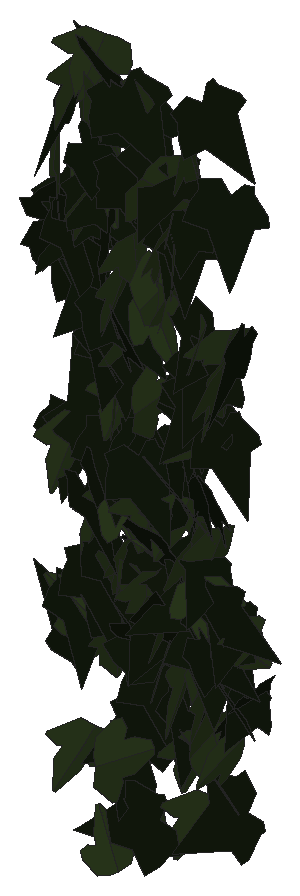
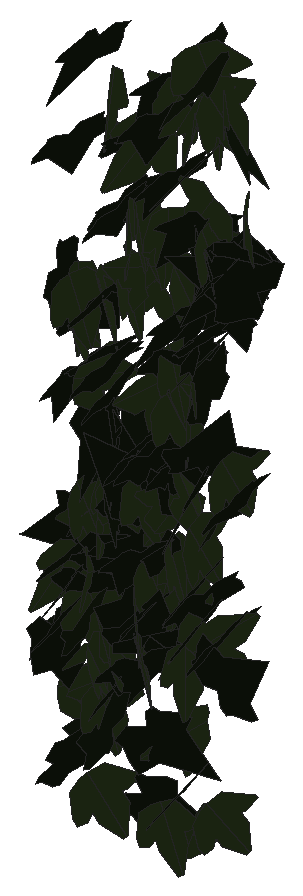
# SketchUp Ruby script. Lengths in inches.
U = 1.inch
M = Sketchup.active_model
def pt(a) = Geom::Point3d.new(a.map { |v| v * U })
def face(e, loops, mat)
  f = e.add_face(loops[0].map { |a| pt(a) })
  loops[1..].each { |l| e.add_face(l.map { |a| pt(a) }).erase! }
  f.material = f.back_material = mat if mat
  f
end
# faces: each face lists its corners as indices into pts; further lists are holes
def faces(e, pts, list, mat = nil) = list.each { |f| face(e, (f[0].is_a?(Array) ? f : [f]).map { |l| l.map { |i| pts[i] } }, mat) }
# xy, xz, yz: faces in a plane at the given z, y or x. An outline is a flat list of corners, or four numbers for a rectangle; further outlines are holes
def ring(l) = l.size == 4 ? [[l[0], l[1]], [l[2], l[1]], [l[2], l[3]], [l[0], l[3]]] : l.each_slice(2).to_a
def flat(e, list, mat, &to3) = list.each { |f| face(e, (f[0].is_a?(Array) ? f : [f]).map { |l| ring(l).map { |u, v| to3.(u, v) } }, mat) }
def xy(e, z, list, mat = nil) = flat(e, list, mat) { |x, y| [x, y, z] }
def xz(e, y, list, mat = nil) = flat(e, list, mat) { |x, z| [x, y, z] }
def yz(e, x, list, mat = nil) = flat(e, list, mat) { |y, z| [x, y, z] }
def lines(e, pts, list) = list.each { |a, b| e.add_line(pt(pts[a]), pt(pts[b])) }
# prism: a flat outline (further loops are holes) pulled along v
def prism(e, loops, v, mat = nil)
  f = face(e, loops, mat); d = Geom::Vector3d.new(v.map { |x| x * U })
  f.pushpull(f.normal.samedirection?(d) ? d.length : -d.length)
end
def box(e, o, s, mat = nil) = prism(e, [[o, [o[0] + s[0], o[1], o[2]], [o[0] + s[0], o[1] + s[1], o[2]], [o[0], o[1] + s[1], o[2]]]], [0, 0, s[2]], mat)
def at(x, y, z, deg = 0) = Geom::Transformation.translation(pt([x, y, z])) * Geom::Transformation.rotation(ORIGIN, Z_AXIS, deg.degrees)
def axes(o, x, y, z) = Geom::Transformation.new([*x, 0, *y, 0, *z, 0, *pt(o).to_a, 1])
def part(name) = M.definitions.add(name)
# library, detail: a bought-in or finely detailed component or shape, given as its bounding box
def library(name, o, s) = part(name).tap { |d| box(d.entities, o, s) }
def detail(e, o, s) = box(e.add_group.entities, o, s)
def put(e, d, t, mat = nil) = e.add_instance(d, t).tap { |i| i.material = mat if mat }
def group(e, t, mat = nil) = e.add_group.tap { |g| g.transformation = t; g.material = mat if mat }.entities
root = M.entities
M.materials.add("efeu1").color = [18, 25, 13]
M.materials.add("efeu2").color = [43, 57, 29]
c1 = part("ivyleaf_9")
p = [[1.54,2.16,1.25],[1.36,2.04,1.19],[-0.21,0.99,0.68],[-0.71,1.11,0.82],[-0.85,0.86,0.67],[-0.8,0.17,0.21],
  [-0.9,-0.01,0.1],[-0.67,-0.16,-0.02],[-0.08,-0.08,-0.05],[-0.03,-0.6,-0.4],[0.65,-0.88,-0.66],[0.83,-0.6,-0.49],
  [1.29,-0.42,-0.43],[1.8125,-0.07,-0.26],[1.21,0.44,0.15]]
faces(c1.entities,p,[[0,1,2,3,4,5,6,7,8,9,10,11,12,13,14]],"efeu1")
c2 = part("ivyleaf_10")
p = [[0,0.5,-0.03],[-0.0625,2.02,-0.43],[-0.19,2.01,-0.46],[-0.54,1.05,-0.29],[-0.52,0.625,-0.18],[-0.83,0.76,-0.28],
  [-1.16,0.64,-0.33],[-1.15,0.33,-0.24],[-0.77,-0.39,0.02],[-0.3,-0.51,0.16],[0.04,-0.48,0.23],[-0.02,2.01,-0.4375],
  [-0.06,2.01,-0.43],[0.04,-0.49,0.23],[0.67,-0.49,0.14],[1.38,0.36,-0.2],[1.375,0.51,-0.24],[0.81,0.65,-0.19],
  [0.62,0.59,-0.15],[0.6,1.09,-0.28],[0.5,1.23,-0.31]]
faces(c2.entities,p,[[0,1,2,3,4,5,6,7,8,9,10],[11,12,0,13,14,15,16,17,18,19,20]],"efeu2")
put(root,c1,axes([522.17,133.86,190.29],[0.49704,-0.38709,-0.5058],[-0.2385,0.4818,-0.60309],[0.59059,0.52034,0.18214]))
put(root,c2,axes([519.06,134.07,182.82],[0.11061,0.72226,0.03],[-0.05424,-0.02197,0.72895],[0.72084,-0.11248,0.05025]))
put(root,c2,axes([519.3,133.52,185.96],[0.08059,-0.14337,-0.86405],[0.35934,0.79672,-0.09868],[0.79875,-0.34396,0.13158]))
put(root,c2,axes([517.37,134.58,194.53],[-0.17439,-0.69901,0.42648],[0.13226,-0.45437,-0.69063],[0.80809,-0.07649,0.20507]))
put(root,c1,axes([517.86,134.49,192.92],[0.40289,-0.6896,0.17223],[0.08138,-0.15191,-0.79864],[0.70611,0.41098,-0.00622]))
put(root,c2,axes([521.91,134.17,191.51],[0.62913,0.42133,0.11867],[0.08795,0.08188,-0.75695],[-0.4288,0.63497,0.01886]))
put(root,c1,axes([519.75,134.29,194.6],[0.10741,-0.71739,-0.34234],[0.00616,0.34619,-0.72352],[0.79486,0.09426,0.05187]))
put(root,c2,axes([518.95,134.53,199.5625],[0.20121,-0.74109,0.28245],[0.09613,-0.26646,-0.76761],[0.78724,0.22195,0.02154]))
put(root,c1,axes([520.43,134.78,203.37],[-0.3338,-0.74643,0.16803],[-0.00432,-0.18148,-0.81477],[0.76509,-0.32668,0.0687]))
put(root,c1,axes([520.19,134.43,184.13],[-0.15629,-0.12747,-0.81514],[-0.62348,-0.52511,0.20166],[-0.54035,0.64277,0.00309]))
put(root,c1,axes([520.42,134.11,194.5625],[0.78632,-0.27011,-0.05779],[-0.05213,0.02613,-0.83139],[0.27126,0.78801,0.00775]))
put(root,c1,axes([517.59,134.72,189.65],[0.05804,-0.8437,0.16627],[0.01144,-0.16588,-0.84569],[0.85985,0.05916,0.00002]))
put(root,c1,axes([521.65,134.83,192.1],[-0.09761,-0.68958,0.36515],[-0.01287,-0.36653,-0.69561],[0.78019,-0.09232,0.03421]))
put(root,c1,axes([522.12,134.17,191.16],[0.13868,-0.13524,-0.79554],[0.62573,0.52773,0.01937],[0.50955,-0.61125,0.19273]))
put(root,c1,axes([517.32,134.57,204.45],[-0.60436,0.19155,-0.52821],[0.47673,-0.23575,-0.63095],[-0.29736,-0.76726,0.062]))
put(root,c1,axes([518.25,133.97,203.38],[0.56318,-0.38083,-0.47393],[-0.17077,0.52092,-0.62152],[0.5835,0.52003,0.27552]))
put(root,c1,axes([519.25,134.31,205.18],[0.0955,-0.69118,-0.44409],[0.14908,0.45424,-0.67492],[0.80791,-0.00212,0.17703]))
put(root,c2,axes([521.65,134.91,195.89],[-0.14462,-0.10083,0.78985],[0.0062,-0.80289,-0.10135],[0.79623,-0.01206,0.14425]))
put(root,c1,axes([521.81,134.81,197.78],[-0.30023,-0.71781,0.15186],[-0.03118,-0.15145,-0.77753],[0.73304,-0.30044,0.02912]))
put(root,c2,axes([518.31,134.51,206.1],[-0.63271,-0.46629,0.31865],[-0.16784,-0.30164,-0.77468],[0.53925,-0.64099,0.13275]))
put(root,c1,axes([518.4,134.875,197.22],[-0.04207,-0.69428,0.40959],[0.11743,-0.41105,-0.6847],[0.7975,0.0239,0.12243]))
put(root,c1,axes([518.49,134.6,198.14],[0.38473,-0.07551,-0.73353],[0.73566,-0.01756,0.38766],[-0.05068,-0.82812,0.05866]))
put(root,c2,axes([522.28,134.9,186.79],[0.00844,-0.18199,0.7631],[0.21291,-0.73397,-0.1774],[0.75506,0.209,0.0415]))
put(root,c2,axes([522.51,134.15,198.11],[0.11036,-0.84178,-0.35734],[-0.03642,0.3556,-0.84893],[0.91376,0.11584,0.00932]))
put(root,c1,axes([521.52,135,196.53],[-0.40109,-0.58474,0.38684],[-0.05831,-0.4163,-0.68974],[0.69869,-0.37042,0.16451]))
put(root,c2,axes([517.65,134.76,205.16],[-0.01384,-0.80711,0.4035],[-0.0046,-0.40348,-0.80722],[0.90234,-0.01444,0.00207]))
put(root,c2,axes([519.91,134.5,199.07],[0.60863,-0.03301,0.65341],[0.65339,-0.01495,-0.60937],[0.03345,0.89283,0.01395]))
put(root,c2,axes([520.73,134.87,188.38],[0.1946,-0.52235,0.60317],[0.33629,-0.50932,-0.54957],[0.72358,0.37719,0.0932]))
put(root,c1,axes([519.81,135.01,189.7],[-0.1723,-0.69422,0.4045],[-0.00224,-0.41328,-0.71024],[0.80347,-0.15002,0.08476]))
put(root,c2,axes([521.98,134.85,197.47],[0.28129,-0.52689,0.55434],[0.28103,-0.47812,-0.59704],[0.71129,0.39727,0.01667]))
put(root,c2,axes([519.53,134.32,200.85],[-0.17105,-0.76245,-0.18321],[0.0524,0.17598,-0.7813],[0.7824,-0.17847,0.01227]))
put(root,c2,axes([518.14,134.57,189.22],[0.47774,0.37209,0.62338],[-0.48753,-0.38852,0.60553],[0.53793,-0.68256,-0.00485]))
put(root,c2,axes([518,134.33,204.92],[-0.69899,0.40267,0.24094],[-0.2738,0.00109,-0.79612],[-0.38109,-0.73935,0.13005]))
put(root,c2,axes([520.36,134.04,203.03],[-0.36919,-0.4983,-0.65806],[0.3572,0.55344,-0.61948],[0.74415,-0.51288,-0.02912]))
put(root,c2,axes([519.77,134.71,190.84],[-0.04253,-0.75345,0.21901],[-0.01041,-0.21877,-0.75464],[0.78456,-0.04374,0.00186]))
put(root,c2,axes([518.98,134.38,191.07],[-0.82566,0.06183,-0.04539],[0.0448,-0.00958,-0.82795],[-0.06226,-0.82685,0.0062]))
put(root,c1,axes([522.6,134.92,198.75],[-0.24296,0.17122,-0.76702],[0.5656,-0.51932,-0.29508],[-0.54565,-0.61454,0.03566]))
put(root,c1,axes([518.0625,134.23,206.23],[0.75048,-0.24329,-0.31092],[-0.25355,0.21488,-0.78015],[0.30262,0.78341,0.11743]))
put(root,c1,axes([521.85,134.72,189.95],[-0.44251,-0.53442,-0.4027],[0.3035,0.26999,-0.6918],[0.59638,-0.53394,0.05325]))
put(root,c1,axes([520.82,135,187.24],[0.06526,-0.7069,0.31374],[0.00111,-0.31477,-0.70945],[0.7734,0.0601,-0.02546]))
put(root,c1,axes([521.51,134.93,190.95],[-0.6297,-0.27747,0.39813],[-0.36798,-0.15219,-0.68808],[0.31636,-0.72929,-0.00788]))
put(root,c1,axes([519.86,134.7,189.11],[0.76999,0.1758,0.2885],[-0.28254,-0.05857,0.78979],[0.18523,-0.82017,0.00544]))
put(root,c2,axes([520.36,134.53,201.18],[0.23735,-0.77855,-0.13077],[-0.02824,0.12809,-0.81386],[0.78895,0.2388,0.0102]))
put(root,c2,axes([521.91,134.55,189.26],[-0.6783,-0.26558,0.32911],[-0.30915,-0.11308,-0.72841],[0.28857,-0.7454,-0.00676]))
put(root,c2,axes([521.33,134.26,204.27],[0.25776,-0.65205,-0.46729],[-0.01694,0.48629,-0.6879],[0.80202,0.21983,0.13566]))
put(root,c2,axes([518.51,134.33,204.65],[-0.26429,0.78796,0.1323],[-0.03739,0.127,-0.83109],[-0.79812,-0.26688,-0.00487]))
put(root,c1,axes([521.66,134.3125,194.59],[0.70794,-0.04043,-0.48017],[-0.4807,0.00016,-0.70873],[0.03355,0.85542,-0.02257]))
put(root,c1,axes([517.38,134.64,199.59],[-0.1731,-0.19482,-0.78981],[0.7122,0.35389,-0.24339],[0.39308,-0.72699,0.09318]))
put(root,c1,axes([521.59,134.28,194.67],[0.36377,0.00093,-0.774],[-0.77274,0.04919,-0.36312],[0.04412,0.85381,0.02176]))
put(root,c1,axes([519.05,134.68,202.67],[0.1887,-0.7555,-0.26525],[0.01469,0.27573,-0.77492],[0.80057,0.17302,0.07674]))
put(root,c1,axes([517.24,134.92,200.49],[0.08651,-0.80557,0.01218],[0.00124,-0.01211,-0.8102],[0.80566,0.08652,-0.00006]))
put(root,c1,axes([522.16,135.14,190.74],[-0.11641,-0.7799,0.28254],[0.04431,-0.29074,-0.7843],[0.82831,-0.09406,0.08166]))
put(root,c2,axes([519.03,134.71,191.6],[0.20873,-0.75785,0.03815],[0.00888,-0.03713,-0.78607],[0.75876,0.20892,-0.00129]))
put(root,c1,axes([518.04,134.78,190.8125],[0.05977,-0.8047,-0.22714],[-0.01716,0.22649,-0.80692],[0.83597,0.06219,-0.00032]))
put(root,c2,axes([521.39,134.34,192.55],[-0.01164,-0.75078,-0.43594],[0.01078,0.43582,-0.75087],[0.8681,-0.01548,0.00348]))
put(root,c2,axes([521.3,134.76,186.71],[-0.22352,-0.72706,0.15668],[-0.02578,-0.15593,-0.76036],[0.74331,-0.22405,0.02074]))
put(root,c2,axes([521.34,134.71,198.52],[0.46789,-0.68621,-0.01716],[-0.00702,0.01598,-0.83054],[0.68639,0.46793,0.00321]))
put(root,c1,axes([521.72,134.85,188.99],[0.48119,-0.58167,0.28923],[0.19079,-0.21752,-0.75486],[0.62096,0.51757,0.0078]))
put(root,c2,axes([519.85,134.79,193.31],[-0.33881,-0.74743,0.17146],[-0.03095,-0.17397,-0.81952],[0.76622,-0.33753,0.04271]))
put(root,c1,axes([522.2,134.95,202.79],[-0.1043,-0.80782,-0.10846],[0.01674,0.1072,-0.81452],[0.8149,-0.1056,0.00285]))
put(root,c1,axes([521.73,134.47,205.55],[0.26748,-0.59476,-0.53681],[-0.10627,0.53459,-0.64527],[0.79411,0.27188,0.09446]))
put(root,c1,axes([522.36,135.32,184.72],[-0.31394,-0.46681,0.63515],[-0.3551,-0.52662,-0.56255],[0.70373,-0.47397,-0.00051]))
put(root,c1,axes([519.53,134.49,192.12],[0.74805,-0.12324,0.3191],[0.31355,-0.05966,-0.7581],[0.13673,0.81108,-0.00728]))
put(root,c2,axes([520.64,134.92,193.16],[-0.31739,-0.62272,0.34803],[-0.11261,-0.33241,-0.69747],[0.70443,-0.33372,0.04531]))
put(root,c2,axes([518.97,134.69,204.72],[0.65571,-0.09204,0.51456],[0.5222,0.07847,-0.65141],[0.02335,0.8298,0.11868]))
put(root,c2,axes([516.52,134.91,202.2],[0.46983,-0.54733,0.40577],[0.40916,-0.16747,-0.69964],[0.5448,0.59778,0.17552]))
put(root,c2,axes([517.98,135.08,192.57],[0.08025,-0.74492,0.4313],[0.15231,-0.41405,-0.74346],[0.84719,0.145,0.09281]))
put(root,c2,axes([519.13,134.39,193.07],[0.35099,0.57622,0.41951],[0.22584,0.35362,-0.67466],[-0.67603,0.4173,-0.00758]))
put(root,c1,axes([518.58,134.59,198.79],[0.31378,-0.67534,-0.46793],[0.01515,0.50556,-0.7195],[0.82147,0.24864,0.192]))
put(root,c1,axes([517.41,135.06,201.09],[-0.69139,-0.39869,-0.02994],[0.02723,0.01271,-0.7981],[0.39888,-0.69192,0.00259]))
put(root,c1,axes([518.24,134.49,194.125],[0.48185,-0.45178,-0.49466],[-0.34866,0.35118,-0.66037],[0.57204,0.59459,0.01418]))
put(root,c1,axes([518.49,135.01,194.53],[-0.15416,-0.76532,-0.13074],[0.03688,0.12592,-0.78061],[0.77553,-0.15812,0.01113]))
put(root,c1,axes([520.4375,135.18,201.61],[-0.11757,-0.802,0.12552],[-0.02555,-0.12311,-0.81054],[0.81136,-0.12009,-0.00733]))
put(root,c1,axes([522.06,134.83,196.02],[0.15573,-0.74503,-0.27025],[-0.06775,0.2619,-0.76104],[0.78963,0.16941,-0.01199]))
put(root,c1,axes([520.04,134.92,188.27],[-0.12074,-0.75737,-0.28282],[0.10296,0.26923,-0.76491],[0.80187,-0.14861,0.05562]))
put(root,c1,axes([517.8,135.36,198.5625],[-0.37482,-0.54248,0.44884],[-0.07396,-0.47533,-0.63626],[0.70019,-0.3406,0.17306]))
put(root,c2,axes([521.51,135.15,190.49],[-0.14747,0.33725,-0.66782],[0.16177,-0.65019,-0.36407],[-0.73044,-0.21209,0.0542]))
put(root,c1,axes([518.26,134.74,189.81],[0.40168,-0.62268,-0.23895],[-0.09578,0.2222,-0.74002],[0.66004,0.41119,0.03803]))
put(root,c1,axes([520.97,135,192.95],[-0.42261,0.20859,-0.65759],[0.6103,-0.24653,-0.47042],[-0.32167,-0.74179,-0.02858]))
put(root,c1,axes([521.24,135.37,198.34],[-0.22232,-0.62429,0.45999],[-0.0342,-0.47016,-0.65463],[0.7747,-0.19991,0.10311]))
put(root,c1,axes([519.98,134.69,193.05],[-0.47991,0.32252,0.60719],[0.41326,-0.45647,0.56909],[0.54947,0.62501,0.10231]))
put(root,c1,axes([517.53,135.17,196.92],[0.20375,-0.39841,0.65952],[0.32181,-0.57584,-0.44727],[0.70009,0.38064,0.01366]))
put(root,c1,axes([519.34,134.95,204.33],[-0.04923,-0.78415,-0.25934],[0.0226,0.25842,-0.78567],[0.82561,-0.05383,0.00604]))
put(root,c1,axes([517.06,134.2,200.73],[-0.01842,-0.05644,-0.837],[-0.14896,0.82412,-0.05229],[0.82557,0.14744,-0.02811]))
put(root,c1,axes([522.58,135.35,188.39],[-0.08677,-0.62892,0.45455],[-0.04137,-0.45299,-0.63465],[0.77488,-0.09461,0.01702]))
put(root,c2,axes([518.77,135.07,196.15],[-0.26274,-0.66612,0.34597],[0.00166,-0.36707,-0.70548],[0.7506,-0.23236,0.12266]))
put(root,c1,axes([520.55,135.14,201.3],[0.02957,-0.82043,0.0385],[-0.00518,-0.03871,-0.82094],[0.82132,0.02929,-0.00656]))
put(root,c1,axes([519.58,135.0625,186.54],[0.04291,0.05635,-0.77252],[-0.35568,-0.68587,-0.06979],[-0.68808,0.35806,-0.0121]))
put(root,c1,axes([518.67,135.02,197.75],[-0.20429,-0.7427,-0.23212],[0.07831,0.21915,-0.7701],[0.77417,-0.21815,0.01665]))
put(root,c2,axes([521.32,135.07,188.02],[0.31258,-0.64138,0.30965],[0.15373,-0.26944,-0.71326],[0.69543,0.34784,0.01849]))
put(root,c2,axes([518.48,134.76,193.28],[0.36207,-0.74021,0.06166],[0.02164,0.07908,0.82225],[-0.74246,-0.35867,0.05404]))
put(root,c2,axes([520.63,134.5,200.88],[0.46335,-0.51135,-0.45805],[-0.09168,0.50157,-0.65269],[0.68035,0.41584,0.224]))
put(root,c1,axes([518.12,134.99,191.13],[0.29657,-0.74638,-0.0655],[-0.01219,0.06563,-0.80304],[0.74915,0.29654,0.01286]))
put(root,c2,axes([521.81,134.23,186.86],[0.08769,-0.20611,0.76803],[-0.27027,0.71896,0.2238],[-0.74786,-0.28399,0.00918]))
put(root,c2,axes([521.65,135.08,192.56],[0.0359,-0.8023,0.25423],[0.04447,-0.2523,-0.80248],[0.84044,0.04762,0.0316]))
put(root,c1,axes([517.88,135.1,201.06],[-0.34191,-0.01316,-0.75416],[0.75135,-0.07885,-0.33926],[-0.06642,-0.82428,0.04449]))
put(root,c2,axes([518.7,134.51,196.15],[0.44212,-0.51866,-0.50472],[-0.13079,0.52445,-0.6535],[0.71179,0.41852,0.19342]))
put(root,c2,axes([517.66,135.04,201.23],[0.12279,-0.78308,0.1817],[0.04455,-0.17689,-0.79248],[0.80264,0.12962,0.01619]))
put(root,c2,axes([517.76,134.86,202.25],[0.66577,-0.04122,0.48485],[0.48601,0.09693,-0.65911],[-0.02404,0.81788,0.10255]))
put(root,c2,axes([518.86,134.94,197.42],[0.02087,-0.80675,0.00868],[-0.0008,-0.00871,-0.80702],[0.8068,0.02086,-0.00102]))
put(root,c1,axes([520.1,134.73,188.71],[-0.69846,-0.39113,0.2691],[0.24304,0.11663,0.80036],[-0.40784,0.73936,0.0161]))
put(root,c2,axes([522.61,134.52,190.19],[-0.21683,-0.52961,-0.55132],[0.29981,0.46825,-0.56772],[0.70324,-0.36292,0.07205]))
put(root,c1,axes([516.76,135.34,194.14],[-0.02633,-0.74368,0.2109],[-0.00334,-0.21091,-0.74413],[0.773,-0.02624,0.00397]))
put(root,c2,axes([520.18,134.74,189.85],[0.28327,-0.66026,-0.3094],[-0.06462,0.30789,-0.7162],[0.72629,0.28491,0.05695]))
put(root,c2,axes([520.32,135.01,199.25],[0.21452,-0.78435,0.05426],[0.01744,-0.05148,-0.81315],[0.78603,0.2152,0.00324]))
put(root,c2,axes([518.54,134.85,188.84],[-0.23084,-0.72927,-0.11946],[0.01757,0.1197,-0.76469],[0.73878,-0.23071,-0.01914]))
put(root,c1,axes([517.55,134.73,188.28],[0.13238,0.01031,0.85113],[-0.65638,0.54964,0.09543],[-0.54192,-0.6632,0.09232]))
put(root,c2,axes([519.98,134.96,188.75],[0.47282,-0.63868,-0.11348],[-0.051,0.10339,-0.79439],[0.64667,0.47513,0.02032]))
put(root,c1,axes([519.76,135.27,194.52],[-0.00515,-0.79459,-0.01398],[-0.00011,0.01399,-0.79461],[0.79472,-0.00514,-0.0002]))
put(root,c1,axes([522.74,134.95,188.29],[-0.30705,0.64426,-0.3801],[0.17376,-0.3382,-0.71362],[-0.72757,-0.35266,-0.01002]))
put(root,c2,axes([521.9375,135.12,198.46],[-0.24098,-0.75874,0.1732],[-0.02675,-0.17314,-0.79565],[0.7778,-0.24103,0.0263]))
put(root,c1,axes([520.61,135.4,196.1],[0.06347,-0.75436,0.21104],[-0.00022,-0.21174,-0.75682],[0.78332,0.06106,-0.01731]))
put(root,c1,axes([520.73,135.21,186.25],[0.5197,-0.53509,0.37932],[0.24908,-0.2867,-0.7457],[0.60677,0.576,-0.01878]))
put(root,c1,axes([517.94,134.93,201.78],[0.04596,-0.61099,-0.5297],[0.1933,0.52347,-0.58704],[0.7852,-0.0931,0.17552]))
put(root,c1,axes([520.83,135.33,196.73],[0.05913,-0.80207,0.0263],[0.0024,-0.0262,-0.80425],[0.8025,0.05917,0.00047]))
put(root,c2,axes([520.05,134.32,199.44],[0.13275,0.27585,-0.84181],[0.30034,0.78678,0.30518],[0.83339,-0.32748,0.02411]))
put(root,c1,axes([519.76,135.14,191.6],[-0.02891,-0.70997,-0.30148],[0.11977,0.2939,-0.70361],[0.76197,-0.07313,0.09916]))
put(root,c2,axes([519.1875,135,184.1],[-0.64054,-0.16917,0.35413],[-0.3366,-0.11173,-0.66221],[0.2018,-0.72333,0.01947]))
put(root,c1,axes([519.34,135.3,194.64],[-0.07655,-0.78421,-0.09647],[-0.00434,0.09734,-0.78782],[0.79011,-0.07545,-0.01367]))
put(root,c2,axes([517.14,135.4,185.06],[-0.28565,-0.54241,0.47693],[-0.05048,-0.49662,-0.59505],[0.7205,-0.24984,0.14739]))
put(root,c2,axes([519.8125,134.36,196.17],[0.00294,0.02601,-0.84155],[0.22589,0.81068,0.02585],[0.81108,-0.22587,-0.00415]))
put(root,c1,axes([516.42,134.79,200.24],[0.27118,-0.04869,0.76965],[0.77097,-0.00217,-0.27178],[0.01823,0.81602,0.0452]))
put(root,c1,axes([518.05,134.94,194.71],[-0.68492,-0.48834,0.22532],[0.1861,0.1271,0.84118],[-0.50459,0.70974,0.00439]))
put(root,c2,axes([521.1,135.32,184.45],[-0.35951,-0.60606,0.39445],[-0.14393,-0.37173,-0.70232],[0.70865,-0.38296,0.05747]))
put(root,c1,axes([519.82,134.78,192.93],[-0.29503,-0.10121,0.8328],[0.83483,0.05168,0.30204],[-0.08277,0.882,0.07787]))
put(root,c1,axes([518.47,135.5625,185.02],[-0.01929,-0.6741,0.36436],[0.05402,-0.36476,-0.67199],[0.76436,0.00877,0.05669]))
